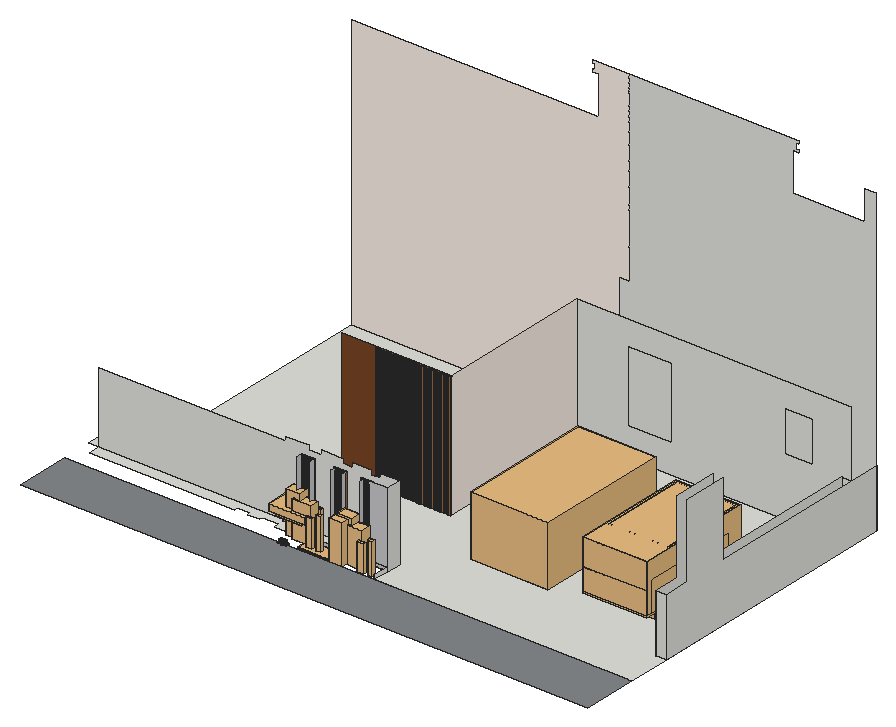
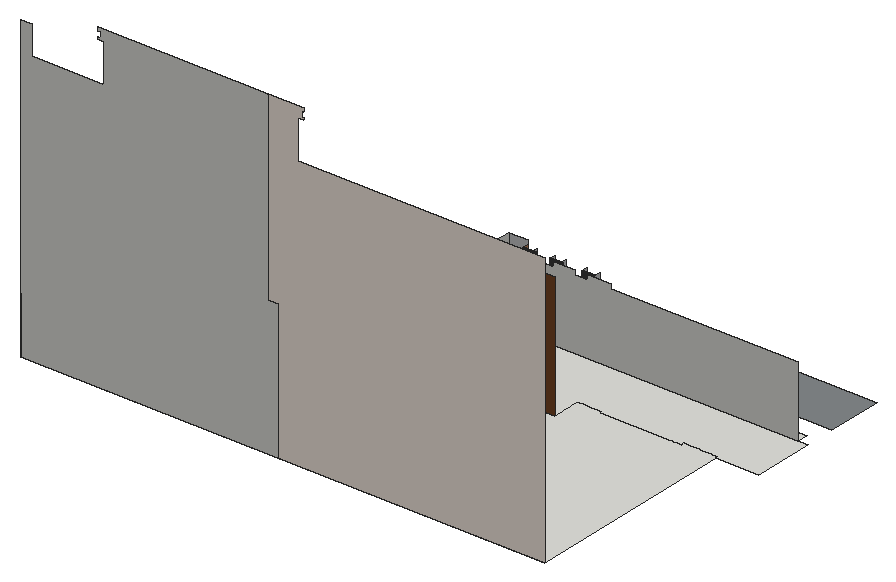
# SketchUp Ruby script. Lengths in inches.
U = 1.inch
M = Sketchup.active_model
def pt(a) = Geom::Point3d.new(a.map { |v| v * U })
def face(e, loops, mat)
  f = e.add_face(loops[0].map { |a| pt(a) })
  loops[1..].each { |l| e.add_face(l.map { |a| pt(a) }).erase! }
  f.material = f.back_material = mat if mat
  f
end
# faces: each face lists its corners as indices into pts; further lists are holes
def faces(e, pts, list, mat = nil) = list.each { |f| face(e, (f[0].is_a?(Array) ? f : [f]).map { |l| l.map { |i| pts[i] } }, mat) }
# xy, xz, yz: faces in a plane at the given z, y or x. An outline is a flat list of corners, or four numbers for a rectangle; further outlines are holes
def ring(l) = l.size == 4 ? [[l[0], l[1]], [l[2], l[1]], [l[2], l[3]], [l[0], l[3]]] : l.each_slice(2).to_a
def flat(e, list, mat, &to3) = list.each { |f| face(e, (f[0].is_a?(Array) ? f : [f]).map { |l| ring(l).map { |u, v| to3.(u, v) } }, mat) }
def xy(e, z, list, mat = nil) = flat(e, list, mat) { |x, y| [x, y, z] }
def xz(e, y, list, mat = nil) = flat(e, list, mat) { |x, z| [x, y, z] }
def yz(e, x, list, mat = nil) = flat(e, list, mat) { |y, z| [x, y, z] }
def lines(e, pts, list) = list.each { |a, b| e.add_line(pt(pts[a]), pt(pts[b])) }
# prism: a flat outline (further loops are holes) pulled along v
def prism(e, loops, v, mat = nil)
  f = face(e, loops, mat); d = Geom::Vector3d.new(v.map { |x| x * U })
  f.pushpull(f.normal.samedirection?(d) ? d.length : -d.length)
end
def box(e, o, s, mat = nil) = prism(e, [[o, [o[0] + s[0], o[1], o[2]], [o[0] + s[0], o[1] + s[1], o[2]], [o[0], o[1] + s[1], o[2]]]], [0, 0, s[2]], mat)
def at(x, y, z, deg = 0) = Geom::Transformation.translation(pt([x, y, z])) * Geom::Transformation.rotation(ORIGIN, Z_AXIS, deg.degrees)
def axes(o, x, y, z) = Geom::Transformation.new([*x, 0, *y, 0, *z, 0, *pt(o).to_a, 1])
def part(name) = M.definitions.add(name)
# library, detail: a bought-in or finely detailed component or shape, given as its bounding box
def library(name, o, s) = part(name).tap { |d| box(d.entities, o, s) }
def detail(e, o, s) = box(e.add_group.entities, o, s)
def put(e, d, t, mat = nil) = e.add_instance(d, t).tap { |i| i.material = mat if mat }
def group(e, t, mat = nil) = e.add_group.tap { |g| g.transformation = t; g.material = mat if mat }.entities
root = M.entities
M.materials.add("Black_matte").color = [7, 7, 7]
M.materials.add("Glass_headlight").color = [127, 127, 127]
M.materials["Glass_headlight"].alpha = 0.29
M.materials.add("[0009_Linen]").color = [250, 240, 230]
M.materials.add("[0022_Maroon]").color = [128, 0, 0]
M.materials.add("[0043_SaddleBrown]").color = [139, 69, 19]
M.materials.add("[0058_Olive]").color = [128, 128, 0]
M.materials.add("[Blacktop Old 01]").color = [132, 136, 139]
M.materials.add("[Polished Concrete New]").color = [200, 200, 203]
M.materials.add("[Wood Floor]").color = [155, 105, 61]
M.materials.add("[Wood Veneer 01]").color = [120, 70, 37]
M.materials.add("[Wood Veneer 02]").color = [190, 128, 91]
c1 = part("Group\#44")
p = [[12.14,1.93,0.52],[12.15,1.96,0.53]]
lines(c1.entities,p,[[0,1]])
detail(c1.entities,[0,0,0],[22.29,22.29,3.9])
c2 = part("EXOTIC-BUSHY-02")
prism(c2.entities,[[[-0.2,0.11,-0.03],[-0.16,0.16,-0.03],[-0.11,0.2,-0.03],[-0.06,0.22,-0.03],[0,0.23,-0.03],[0.06,0.22,-0.03],[0.11,0.2,-0.03],[0.16,0.16,-0.03],[0.2,0.11,-0.03],[0.22,0.06,-0.03],[0.23,0,-0.03],[0.22,-0.06,-0.03],[0.2,-0.11,-0.03],[0.16,-0.16,-0.03],[0.11,-0.2,-0.03],[0.06,-0.22,-0.03],[0,-0.23,-0.03],[-0.06,-0.22,-0.03],[-0.11,-0.2,-0.03],[-0.16,-0.16,-0.03],[-0.2,-0.11,-0.03],[-0.22,-0.06,-0.03],[-0.23,0,-0.03],[-0.22,0.06,-0.03]]],[0,0,12.79],"[0043_SaddleBrown]")
put(c2.entities,c1,axes([-11.15,-11.15,16.66],[1,0,0],[0,1,0],[0,0,-1]))
put(c2.entities,c1,axes([-7.91,-7.91,13.14],[0.71,0,0],[0,0.71,0],[0,0,-0.71]))
put(c2.entities,c1,axes([-5.11,-5.11,9.7],[0.4588,0,0],[0,0.4588,0],[0,0,-0.4588]))
c3 = library("EXOTIC-BAMBOO-TOO",[-9.25,-15.15,0],[30.31,37.46,85.46])
c4 = part("Group\#46")
p = [[0.46,5.4,1.48],[0.55,4.86,1.35],[0.68,4.33,1.23],[0.85,3.8,1.12],[1.04,3.28,1.02],[1.28,2.78,0.93],
  [1.54,2.29,0.84],[1.84,1.82,0.77],[2.17,1.36,0.71],[2.52,0.93,0.66],[2.91,0.52,0.62],[2.91,0,0.48],
  [2.47,0.44,0.52],[2.06,0.9,0.56],[1.68,1.39,0.625],[1.34,1.9,0.7],[1.03,2.43,0.79],[0.76,2.98,0.89],
  [0.53,3.55,1],[0.34,4.13,1.12],[0.19,4.72,1.25],[0.09,5.3125,1.39],[0.02,5.91,1.54],[0,6.51,1.69],
  [0.02,6.88,1.8],[0.1,7.24,1.91],[0.22,7.59,2.02],[0.39,7.92,2.14],[0.6,8.22,2.26],[0.85,8.49,2.38],
  [1.14,8.72,2.49],[1.45,8.91,2.6],[1.8,9.0625,2.71],[2.16,9.17,2.8],[2.53,9.22,2.88],[2.91,9.23,2.95],
  [2.91,4.61,1.72],[2.68,3.89,1.48],[2.18,2.26,0.95],[2.59,5.625,1.93],[1.61,4.02,1.32],[2.34,6.73,2.18],
  [1.25,5.66,1.69],[2.4,7.87,2.5],[1.14,7.72,2.22],[2.4375,8.83,2.76],[2.16,8.77,2.69],[1.89,8.68,2.62],
  [1.625,8.56,2.54],[1.39,8.42,2.46],[1.16,8.24,2.37],[0.97,8.04,2.28],[0.79,7.82,2.19],[0.65,7.58,2.1],
  [0.54,7.32,2.01],[0.45,7.05,1.92],[0.4,6.78,1.84],[0.39,6.49,1.76],[0.41,5.95,1.62],[5.79,6.88,1.8],
  [5.82,6.51,1.69],[5.79,5.91,1.54],[5.73,5.3125,1.39],[5.625,4.72,1.25],[5.48,4.13,1.12],[5.29,3.55,1],
  [5.06,2.98,0.89],[4.79,2.43,0.79],[4.48,1.9,0.7],[4.14,1.39,0.625],[3.76,0.9,0.56],[3.35,0.44,0.52],
  [3.29,0.93,0.66],[3.65,1.36,0.71],[3.98,1.82,0.77],[4.27,2.29,0.84],[4.54,2.78,0.93],[4.77,3.28,1.02],
  [4.97,3.8,1.12],[5.13,4.33,1.23],[5.26,4.86,1.35],[5.35,5.4,1.48],[5.41,5.95,1.62],[5.43,6.49,1.76],
  [5.41,6.78,1.84],[5.36,7.05,1.92],[5.28,7.32,2.01],[5.16,7.58,2.1],[5.02,7.82,2.19],[4.85,8.04,2.28],
  [4.65,8.24,2.37],[4.43,8.42,2.46],[4.1875,8.56,2.54],[3.93,8.68,2.62],[3.66,8.77,2.69],[3.38,8.83,2.76],
  [4.67,7.72,2.22],[3.41,7.87,2.5],[4.5625,5.66,1.69],[3.47,6.73,2.18],[4.21,4.02,1.32],[3.23,5.625,1.93],
  [3.64,2.26,0.95],[3.13,3.89,1.48],[3.29,9.22,2.88],[3.66,9.17,2.8],[4.02,9.0625,2.71],[4.36,8.91,2.6],
  [4.68,8.72,2.49],[4.96,8.49,2.38],[5.21,8.22,2.26],[5.43,7.92,2.14],[5.59,7.59,2.02],[5.72,7.24,1.91],
  [2.91,14.34,0]]
faces(c4.entities,p,[[0,1,2,3,4,5,6,7,8,9,10,11,12,13,14,15,16,17,18,19,20,21,22,23,24,25,26,27,28,29,30,31,32,33,34,35,36,10,37,38,39,40,41,42,43,44,45,46,47,48,49,50,51,52,53,54,55,56,57,58],[59,60,61,62,63,64,65,66,67,68,69,70,71,11,10,72,73,74,75,76,77,78,79,80,81,82,83,84,85,86,87,88,89,90,91,92,93,94,95,96,97,98,99,100,101,102,103,10,36,35,104,105,106,107,108,109,110,111,112,113]],"[0022_Maroon]")
faces(c4.entities,p,[[43,42,41,40,39,38,37,10,9,8,7,6,5,4,3,2,1,0,58,57,56,55,54,53,52,51,50,49,48,47,46,45,44],[99,98,97,96,95,94,93,92,91,90,89,88,87,86,85,84,83,82,81,80,79,78,77,76,75,74,73,72,10,103,102,101,100]],"[0058_Olive]")
lines(c4.entities,p,[[35,114]])
c5 = part("EXOTIC-CROTON")
p = [[0,0,13.11],[0,0,0],[0,0,17.6]]
lines(c5.entities,p,[[0,1],[0,2]])
put(c5.entities,c4,at(-2.91,-14.34,9.43),"[0058_Olive]")
put(c5.entities,c4,at(-13.875,-4.65,9.43,-60),"[0058_Olive]")
put(c5.entities,c4,at(-10.97,9.69,9.43,-120),"[0058_Olive]")
put(c5.entities,c4,at(2.91,14.34,9.43,180),"[0058_Olive]")
put(c5.entities,c4,at(13.875,4.65,9.43,120),"[0058_Olive]")
put(c5.entities,c4,at(10.97,-9.69,9.43,60),"[0058_Olive]")
put(c5.entities,c4,axes([-3.96,11.79,13.11],[-0.73612,-0.425,0],[0.425,-0.73612,0],[0,0,0.85]),"[0058_Olive]")
put(c5.entities,c4,axes([8.24,9.32,13.11],[-0.73612,0.425,0],[-0.425,-0.73612,0],[0,0,0.85]),"[0058_Olive]")
put(c5.entities,c4,axes([3.96,-11.79,13.11],[0.73612,0.425,0],[-0.425,0.73612,0],[0,0,0.85]),"[0058_Olive]")
put(c5.entities,c4,axes([-8.24,-9.32,13.11],[0.73612,-0.425,0],[0.425,0.73612,0],[0,0,0.85]),"[0058_Olive]")
put(c5.entities,c4,axes([12.19,-2.47,13.11],[0,0.85,0],[-0.85,0,0],[0,0,0.85]),"[0058_Olive]")
put(c5.entities,c4,axes([-12.19,2.47,13.11],[0,-0.85,0],[0.85,0,0],[0,0,0.85]),"[0058_Olive]")
put(c5.entities,c4,axes([1.98,9.75,17.6],[-0.68,0,0],[0,-0.68,0],[0,0,0.68]),"[0058_Olive]")
put(c5.entities,c4,axes([7.46,-6.59,17.6],[0.34,0.5889,0],[-0.5889,0.34,0],[0,0,0.68]),"[0058_Olive]")
put(c5.entities,c4,axes([9.4375,3.16,17.6],[-0.34,0.5889,0],[-0.5889,-0.34,0],[0,0,0.68]),"[0058_Olive]")
put(c5.entities,c4,axes([-9.4375,-3.16,17.6],[0.34,-0.5889,0],[0.5889,0.34,0],[0,0,0.68]),"[0058_Olive]")
put(c5.entities,c4,axes([-7.46,6.59,17.6],[-0.34,-0.5889,0],[0.5889,-0.34,0],[0,0,0.68]),"[0058_Olive]")
put(c5.entities,c4,axes([-1.98,-9.75,17.6],[0.68,0,0],[0,0.68,0],[0,0,0.68]),"[0058_Olive]")
c6 = part("Group\#2")
xy(c6.entities,0,[[0,0,1.85,1.85],[2.64,0,4.49,1.85],[5.28,0,7.125,1.85],[7.91,0,9.76,1.85],[10.55,0,12.4,1.85],
  [13.1875,0,15.04,1.85],[15.83,0,17.68,1.85],[18.46,0,20.31,1.85],[21.1,0,22.95,1.85]],"[Wood Floor]")
g1 = group(c6.entities,at(0,0,0))
xy(g1,112.2,[[0,0,1.85,1.85],[2.64,0,4.49,1.85],[5.28,0,7.125,1.85],[7.91,0,9.76,1.85],[10.55,0,12.4,1.85],
  [13.1875,0,15.04,1.85],[15.83,0,17.68,1.85],[18.46,0,20.31,1.85],[21.1,0,22.95,1.85]],"[Wood Floor]")
xz(g1,0,[[0,0,1.85,112.2],[2.64,0,4.49,112.2],[5.28,0,7.125,112.2],[7.91,0,9.76,112.2],[10.55,0,12.4,112.2],
  [13.1875,0,15.04,112.2],[15.83,0,17.68,112.2],[18.46,0,20.31,112.2],[21.1,0,22.95,112.2]],"[Wood Floor]")
xz(g1,1.85,[[0,0,1.85,112.2],[2.64,0,4.49,112.2],[5.28,0,7.125,112.2],[7.91,0,9.76,112.2],[10.55,0,12.4,112.2],
  [13.1875,0,15.04,112.2],[15.83,0,17.68,112.2],[18.46,0,20.31,112.2],[21.1,0,22.95,112.2]],"[Wood Floor]")
yz(g1,0,[[0,0,1.85,112.2]],"[Wood Floor]")
yz(g1,1.85,[[0,0,1.85,112.2]],"[Wood Floor]")
yz(g1,2.64,[[0,0,1.85,112.2]],"[Wood Floor]")
yz(g1,4.49,[[0,0,1.85,112.2]],"[Wood Floor]")
yz(g1,5.28,[[0,0,1.85,112.2]],"[Wood Floor]")
yz(g1,7.125,[[0,0,1.85,112.2]],"[Wood Floor]")
yz(g1,7.91,[[0,0,1.85,112.2]],"[Wood Floor]")
yz(g1,9.76,[[0,0,1.85,112.2]],"[Wood Floor]")
yz(g1,10.55,[[0,0,1.85,112.2]],"[Wood Floor]")
yz(g1,12.4,[[0,0,1.85,112.2]],"[Wood Floor]")
yz(g1,13.1875,[[0,0,1.85,112.2]],"[Wood Floor]")
yz(g1,15.04,[[0,0,1.85,112.2]],"[Wood Floor]")
yz(g1,15.83,[[0,0,1.85,112.2]],"[Wood Floor]")
yz(g1,17.68,[[0,0,1.85,112.2]],"[Wood Floor]")
yz(g1,18.46,[[0,0,1.85,112.2]],"[Wood Floor]")
yz(g1,20.31,[[0,0,1.85,112.2]],"[Wood Floor]")
yz(g1,21.1,[[0,0,1.85,112.2]],"[Wood Floor]")
yz(g1,22.95,[[0,0,1.85,112.2]],"[Wood Floor]")
c7 = library("EXOTIC-BAMBOO",[-8.14,-8.14,0],[38.48,34.74,73.65])
c8 = library("EXOTIC-BULLRUSH",[-0.59,-0.59,-0.94],[7.09,7.09,64.29])
c9 = library("EXOTIC-PEONY",[-0.63,-0.48,-0.08],[13.23,10.24,55.71])
c10 = library("EXOTIC-AMAZON-LILY",[-1.1,-0.12,0],[60.56,66.69,1.97])
c11 = library("EXOTIC-RED-POKER\#1",[-1.18,-1.18,0],[10.24,10.24,66.04])
c12 = library("EXOTICA-CAT-TAIL",[-18.64,-20.64,0],[26.41,31.25,82.25])
c13 = library("2016+Honda+Civic+LX+Sedan",[0.01,0.03,0.02],[16.17,34.46,10.62])
c14 = library("Wheel1",[-0.22,0.28,-1.22],[12.14,34.32,34.67])
c15 = library("Group\#51",[0,0,0],[81,26.91,31.48])
c16 = library("Group\#50",[0,-11.74,0],[75.48,151.34,31.8125])
c17 = library("Group\#49",[0,0,0],[59.24,11.61,17.61])
c18 = library("Group\#52",[0,0,0],[83.57,167.11,42.22])
c19 = library("Group\#53",[0,0,0],[97.91,11.39,8.3])
c20 = library("Group\#54",[0,0,0],[82.49,206.98,67.77])
c21 = library("Group\#55",[0,0,0],[82.02,206.91,71.71])
c22 = part("l405 Vogue 2013")
put(c22.entities,c14,axes([23.09,177.11,0.71],[-1.08,0,0],[0,-1,0],[0,0,1]))
put(c22.entities,c14,axes([83.66,53.48,1.89],[1.08,0,0],[0,-1,0],[0,0,1]))
put(c22.entities,c14,axes([23.09,53.48,1.89],[-1.08,0,0],[0,-1,0],[0,0,1]))
put(c22.entities,c14,axes([83.66,177.11,0.71],[1.08,0,0],[0,-1,0],[0,0,1]))
put(c22.entities,c15,axes([97.16,27.0625,11.6],[-1.08,0,0],[0,-1,0],[0,0,1]))
put(c22.entities,c16,axes([94.18,192.03,48.94],[-1.08,0,0],[0,-1,0],[0,0,1]),"Glass_headlight")
put(c22.entities,c17,axes([85.41,206.68,30.35],[-1.08,0,0],[0,-1,0],[0,0,1]))
put(c22.entities,c18,axes([98.55,177.66,12.76],[-1.08,0,0],[0,-1,0],[0,0,1]))
put(c22.entities,c19,axes([106.29,85.5,53.72],[-1.08,0,0],[0,-1,0],[0,0,1]))
put(c22.entities,c20,axes([97.96,207.84,12.8],[-1.08,0,0],[0,-1,0],[0,0,1]))
put(c22.entities,c21,axes([97.7,207.32,9.05],[-1.08,0,0],[0,-1,0],[0,0,1]))
c23 = part("2013 Land Rover Range Rover l405")
put(c23.entities,c22,axes([0,0,0],[1,0,0],[0,1.03,0],[0,0,1]),"Black_matte")
c24 = part("2014+Range+Rover+l405+UK-version+ISA")
put(c24.entities,c23,at(0,0,0),"Black_matte")
xy(root,0,[[641.18,114.25,1176.625,114.25,1176.625,203.31,1155.46,203.31,1155.46,683.93,606.93,683.93,606.93,359.87,378.25,359.87,378.25,300.43,328.15,300.43,328.15,304.24,160.07,304.24,160.07,298.43,88.9375,298.43,88.9375,304.24,0,304.24,0,178.37,643.56,178.37,643.56,148.8],[641.18,114.25,643.56,148.8,641.18,148.8],[408.3,148.8,454.65,148.8,454.65,160.36,481.51,160.36,481.51,148.8,525.01,148.8,525.01,160.36,547.38,160.36,547.38,148.8,584.28,148.8,584.28,160.36,603.91,160.36,603.91,148.8,643.56,148.8,643.56,178.37,20.0625,178.37,20.0625,153.99,321.78,153.99,321.78,160.36,347.76,160.36,347.76,153.99,373.77,153.99,373.77,160.36,408.3,160.36],[1155.46,203.31,1176.625,203.31,1176.625,747.375,88.9375,747.375,88.9375,298.43,160.07,298.43,160.07,304.24,328.15,304.24,328.15,300.43,378.25,300.43,378.25,359.87,606.93,359.87,606.93,683.93,1155.46,683.93]])
xy(root,0,[[0,0,1176.625,114.25],[454.65,148.8,481.51,160.36],[525.01,148.8,547.38,160.36],[584.28,148.8,603.91,160.36]],"[Blacktop Old 01]")
xz(root,148.8,[[454.65,0,481.51,0.6875],[525.01,0,547.38,0.6875],[584.28,0,603.91,0.6875],[454.65,0.6875,481.51,7.8125],[525.01,0.6875,547.38,7.8125],
  [584.28,0.6875,603.91,7.8125]])
xz(root,148.8,[[481.51,0,525.01,0.6875],[547.38,0,584.28,0.6875],[603.91,0,641.18,0.6875],[641.18,0,643.56,0,643.56,155.375,603.91,155.375,603.91,7.8125,641.18,7.8125],[481.51,0.6875,525.01,7.8125],
  [547.38,0.6875,584.28,7.8125],[603.91,0.6875,641.18,7.8125]],"[Polished Concrete New]")
xz(root,160.36,[[454.65,0,481.51,146.4375],[525.01,0,547.38,146.4375],[584.28,0,603.91,146.4375]],"[Wood Veneer 02]")
xz(root,178.37,[[20.0625,0,20.0625,146.4375,408.3,146.4375,408.3,155.375,454.65,155.375,454.65,146.4375,481.51,146.4375,481.51,155.375,525.01,155.375,525.01,146.4375,547.38,146.4375,547.38,155.375,584.28,155.375,584.28,146.4375,603.91,146.4375,603.91,155.375,643.56,155.375,643.56,0]])
xz(root,203.31,[[1155.46,0,1176.625,119.9375]])
xz(root,359.87,[[378.25,0,606.93,258.1]],"[Wood Veneer 01]")
xz(root,683.93,[[[606.93,0,1155.46,0,1155.46,119.9375,1174.71,119.9375,1174.71,258.1,606.93,258.1],[711.72,59.63,803.59,208.29],[1036.79,120.97,1094.73,206.28]]])
xz(root,747.375,[[643.56,0,643.56,285.125,664.06,285.125,664.06,668.375,1016.65,668.375,1016.65,662.48,1009.71,662.48,1009.71,651.03,1016.65,651.03,1016.65,646.01,1002.71,646.01,1002.71,566.3125,1153.77,566.3125,1153.77,626.3125,1174.71,626.3125,1174.71,119.9375,1176.625,119.9375,1176.625,0]])
xz(root,747.375,[[88.9375,0,88.9375,566.3125,601.41,566.3125,601.41,646.01,588.47,646.01,588.47,651.03,592.41,651.03,592.41,662.48,588.47,662.48,588.47,668.375,664.06,668.375,664.06,285.125,643.56,285.125,643.56,0]],"[0009_Linen]")
yz(root,454.65,[[148.8,0,160.36,146.4375]],"[Polished Concrete New]")
yz(root,481.51,[[148.8,0,160.36,146.4375]],"[Polished Concrete New]")
yz(root,525.01,[[148.8,0,160.36,146.4375]],"[Polished Concrete New]")
yz(root,547.38,[[148.8,0,160.36,146.4375]],"[Polished Concrete New]")
yz(root,584.28,[[148.8,0,160.36,146.4375]],"[Polished Concrete New]")
yz(root,603.91,[[148.8,0,160.36,146.4375]],"[Wood Veneer 02]")
yz(root,606.93,[[359.87,0,683.93,258.1]],"[0009_Linen]")
yz(root,641.18,[[114.25,0,148.8,0,148.8,0.6875,118.08,0.6875,118.08,7.8125,114.25,7.8125]])
yz(root,643.56,[[148.8,0,178.37,155.375]])
yz(root,1155.46,[[203.31,0,203.31,119.9375,256.56,119.9375,256.56,272.3125,349.72,272.3125,349.72,119.9375,683.93,119.9375,683.93,0]])
yz(root,1176.625,[[203.31,0,747.375,0,747.375,119.9375,349.72,119.9375,349.72,272.3125,256.56,272.3125,256.56,119.9375,203.31,119.9375]])
p = [[641.18,114.25,0],[643.56,148.8,0],[643.56,148.8,7.8125],[641.18,114.25,7.8125]]
faces(root,p,[[0,1,2,3]])
put(root,c2,axes([448.87,150.94,-2.83],[3.38,0,0],[0,1.93843,0],[0,0,3.38]))
put(root,c3,axes([447.21,148.16,0.6875],[1,0,0],[0,0.5735,0],[0,0,1]))
put(root,c5,axes([454.41,112.96,-5.96],[0.783,0,0],[0,0.44905,0],[0,0,0.783]))
put(root,c6,axes([456.2,159.42,0],[1.13172,0,0],[0,0.84111,0],[0,0,1.30509]))
put(root,c7,axes([462.92,140.34,0.6875],[1,0,0],[0,0.5735,0],[0,0,1]))
put(root,c6,axes([452.34,355.95,0],[2.12,0,0],[0,2.12,0],[0,0,2.2896]))
put(root,c8,axes([491.34,156.95,-2.89],[1,0,0],[0,0.5735,0],[0,0,1]))
put(root,c9,axes([489.21,128.23,0.6875],[1,0,0],[0,0.5735,0],[0,0,1]))
put(root,c10,axes([478.69,121.75,-2.89],[1,0,0],[0,0.5735,0],[0,0,1]))
put(root,c11,axes([510.21,134.37,0.6875],[0,-0.5735,0],[1,0,0],[0,0,1]))
put(root,c6,axes([497.65,355.95,0],[2.12,0,0],[0,2.12,0],[0,0,2.2896]))
put(root,c6,axes([522.07,159.42,0],[1.13172,0,0],[0,0.84111,0],[0,0,1.30509]))
put(root,c12,axes([565.04,129.17,-2.89],[1,0,0],[0,0.5735,0],[0,0,1]))
put(root,c3,axes([559.39,141.7,-2.89],[1,0,0],[0,0.5735,0],[0,0,1]))
put(root,c6,axes([545.9,355.95,0],[2.65,0,0],[0,2.12,0],[0,0,2.2896]))
put(root,c7,axes([575.1,133.88,-2.89],[1,0,0],[0,0.5735,0],[0,0,1]))
put(root,c6,axes([577.93,158.81,0],[1.13172,0,0],[0,0.84111,0],[0,0,1.30509]))
put(root,c9,axes([601.4,121.77,-2.89],[1,0,0],[0,0.5735,0],[0,0,1]))
put(root,c11,axes([622.39,127.9,-2.89],[0,-0.5735,0],[1,0,0],[0,0,1]))
put(root,c13,axes([722.32,263.8,-0.08],[9.93409,0,0],[0,8.0765,0],[0,0,11.71093]))
put(root,c24,axes([935.17,271.5,0.23],[1.5,0,0],[0,1.1305,0],[0,0,1.45547]))
